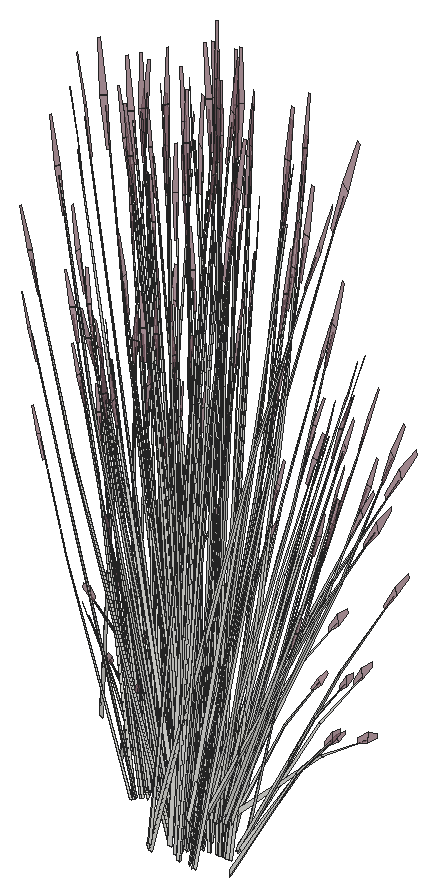
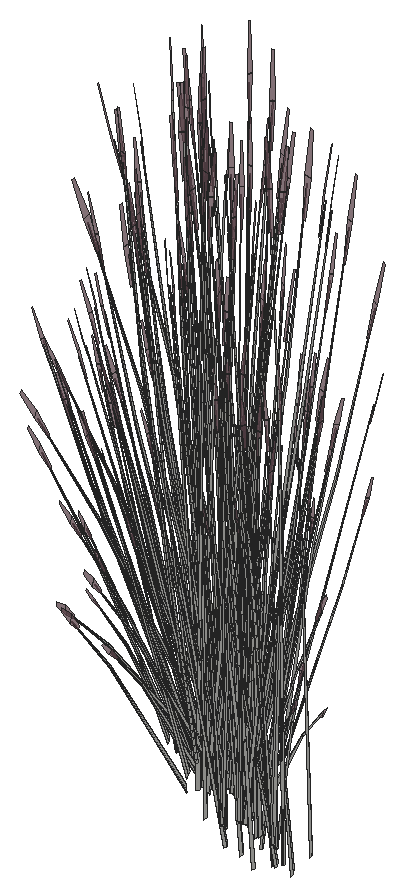
# SketchUp Ruby script. Lengths in inches.
U = 1.inch
M = Sketchup.active_model
def pt(a) = Geom::Point3d.new(a.map { |v| v * U })
def face(e, loops, mat)
  f = e.add_face(loops[0].map { |a| pt(a) })
  loops[1..].each { |l| e.add_face(l.map { |a| pt(a) }).erase! }
  f.material = f.back_material = mat if mat
  f
end
# faces: each face lists its corners as indices into pts; further lists are holes
def faces(e, pts, list, mat = nil) = list.each { |f| face(e, (f[0].is_a?(Array) ? f : [f]).map { |l| l.map { |i| pts[i] } }, mat) }
# xy, xz, yz: faces in a plane at the given z, y or x. An outline is a flat list of corners, or four numbers for a rectangle; further outlines are holes
def ring(l) = l.size == 4 ? [[l[0], l[1]], [l[2], l[1]], [l[2], l[3]], [l[0], l[3]]] : l.each_slice(2).to_a
def flat(e, list, mat, &to3) = list.each { |f| face(e, (f[0].is_a?(Array) ? f : [f]).map { |l| ring(l).map { |u, v| to3.(u, v) } }, mat) }
def xy(e, z, list, mat = nil) = flat(e, list, mat) { |x, y| [x, y, z] }
def xz(e, y, list, mat = nil) = flat(e, list, mat) { |x, z| [x, y, z] }
def yz(e, x, list, mat = nil) = flat(e, list, mat) { |y, z| [x, y, z] }
def lines(e, pts, list) = list.each { |a, b| e.add_line(pt(pts[a]), pt(pts[b])) }
# prism: a flat outline (further loops are holes) pulled along v
def prism(e, loops, v, mat = nil)
  f = face(e, loops, mat); d = Geom::Vector3d.new(v.map { |x| x * U })
  f.pushpull(f.normal.samedirection?(d) ? d.length : -d.length)
end
def box(e, o, s, mat = nil) = prism(e, [[o, [o[0] + s[0], o[1], o[2]], [o[0] + s[0], o[1] + s[1], o[2]], [o[0], o[1] + s[1], o[2]]]], [0, 0, s[2]], mat)
def at(x, y, z, deg = 0) = Geom::Transformation.translation(pt([x, y, z])) * Geom::Transformation.rotation(ORIGIN, Z_AXIS, deg.degrees)
def axes(o, x, y, z) = Geom::Transformation.new([*x, 0, *y, 0, *z, 0, *pt(o).to_a, 1])
def part(name) = M.definitions.add(name)
# library, detail: a bought-in or finely detailed component or shape, given as its bounding box
def library(name, o, s) = part(name).tap { |d| box(d.entities, o, s) }
def detail(e, o, s) = box(e.add_group.entities, o, s)
def put(e, d, t, mat = nil) = e.add_instance(d, t).tap { |i| i.material = mat if mat }
def group(e, t, mat = nil) = e.add_group.tap { |g| g.transformation = t; g.material = mat if mat }.entities
root = M.entities
M.materials.add("LightPink_Translucent").color = [144, 107, 117]
M.materials["LightPink_Translucent"].alpha = 0.75
c1 = part("blade")
p = [[2.15,0.21,22],[0,0.17,0],[0.09,0.45,0],[2.18,0.31,22],[2.29,0.31,22],[0.38,0.45,0],
  [2.48,0.24,33],[2.49,0.24,33],[2.48,0.22,33]]
faces(c1.entities,p,[[0,1,2,3],[4,5,2,3],[6,3,4,7],[8,0,3,6]])
c2 = part("seeds")
p = [[0.3,-0.1,1.38],[-0.01,-0.03,1.59],[-0.01,-0.03,0.03],[0.14,-0.07,-0.07],[0.29,-0.03,3],[0.15,0.01,3.11]]
faces(c2.entities,p,[[0,1,2,3],[1,0,4,5]],"LightPink_Translucent")
c3 = part("blade with seeds")
put(c3.entities,c1,at(0,0,0))
put(c3.entities,c2,axes([2.4,0.25,30.99],[1.5799,-0.05474,1.17369],[-0.12525,1.92788,0.29478],[-0.07173,-0.02425,1.56792]))
put(root,c3,axes([688.24,330.9,391.83],[0,-0.66065,0],[0.81352,0,0],[0,0,1.48949]))
put(root,c3,axes([689.22,329.375,392.06],[-0.60889,-0.28548,0.4121],[0.36394,-0.51192,0],[0.13868,0.06502,1.30728]))
put(root,c3,axes([690.42,331.38,394.13],[0.57168,-0.25217,-0.58968],[0.3186,0.51908,0.07116],[0.27622,-0.05897,0.83415]))
put(root,c3,axes([686.79,331.71,391.71],[-0.67676,-0.09361,-0.51753],[0.14281,-0.57742,-0.13583],[-0.20196,-0.06997,1.14236]))
put(root,c3,axes([687.85,330.48,391.96],[-0.53943,0.51816,0.37976],[-0.64086,-0.4574,0.14902],[0.13005,-0.05171,1.31851]))
put(root,c3,axes([688.44,331.41,391.91],[-0.60515,-0.49144,-0.05089],[0.60552,-0.49174,0],[-0.02113,-0.01716,1.45724]))
put(root,c3,axes([686.92,329.63,392.05],[-0.18794,0.56744,0.14643],[-0.68774,-0.16058,0.29122],[0.1188,-0.00276,1.33138]))
put(root,c3,axes([690.33,331.48,394.19],[-0.54068,-0.15928,0.29394],[0.1577,-0.46469,-0.37948],[0.21769,-0.04261,0.72609]))
put(root,c3,axes([684.67,330.63,393.93],[0.18381,-0.5206,0.39842],[0.60429,0.17802,0.32852],[-0.23764,0.03129,0.82444]))
put(root,c3,axes([686.63,330.09,391.32],[-0.64037,0.22859,1.07011],[-0.20382,-0.65589,0.4158],[0.39323,0.01091,1.21713]))
put(root,c3,axes([688.35,330.26,392.17],[0.12551,-0.50956,0.12018],[0.6132,0.08845,-0.34318],[0.1116,0.05232,1.05198]))
put(root,c3,axes([684.625,330.49,393.93],[-0.23895,-0.38931,0.05337],[0.43573,-0.19055,0.42015],[-0.19208,0.0376,0.64067]))
put(root,c3,axes([687.29,331.47,391.96],[0.82229,0.1203,0.37976],[-0.16734,0.67942,0.14902],[-0.12017,-0.06561,1.31851]))
put(root,c3,axes([691.63,330.98,391.24],[-0.034,-0.08668,1.46364],[0.23582,-0.50706,-0.2236],[0.23788,-0.00729,0.24931]))
put(root,c3,axes([688.09,330.4,392.26],[-0.39083,-0.47924,0.37133],[0.59199,-0.33747,-0.17871],[0.12647,0.0593,1.19224]))
put(root,c3,axes([686.07,332.59,391.68],[-0.15283,-0.49751,-0.25712],[0.60696,-0.14127,0.25712],[-0.12236,-0.05737,1.15348]))
put(root,c3,axes([686.85,332.56,392.05],[0.6991,-0.15154,0.14643],[0.17263,0.56398,0.29122],[-0.06235,-0.08217,1.33138]))
put(root,c3,axes([688.29,330.43,392.21],[0.65687,-0.37907,-0.24149],[0.43681,0.53562,-0.41502],[0.16207,0.0544,1.32557]))
put(root,c3,axes([690.9,331.43,393.76],[0.54068,0.15928,-0.29394],[-0.1577,0.46469,0.37948],[0.21769,-0.04261,0.72609]))
put(root,c3,axes([685.9,332.8,391.67],[-0.60889,-0.28548,-0.4121],[0.36394,-0.51192,0],[-0.13868,-0.06502,1.30728]))
put(root,c3,axes([689.95,329.42,391.67],[0.60889,0.28548,-0.4121],[-0.36394,0.51192,0],[0.13868,0.06502,1.30728]))
put(root,c3,axes([688.79,331.05,391.83],[0.72788,0,0],[0,0.59111,0],[0,0,1.48078]))
put(root,c3,axes([687.56,331.79,392.21],[-0.65687,0.37907,-0.24149],[-0.43681,-0.53562,-0.41502],[-0.16207,-0.0544,1.32557]))
put(root,c3,axes([689,329.66,392.05],[-0.6991,0.15154,0.14643],[-0.17263,-0.56398,0.29122],[0.06235,0.08217,1.33138]))
put(root,c3,axes([689.43,330.85,393.22],[-0.26985,0.01293,1.42242],[0.17902,-0.56047,0.11501],[0.38456,0.03467,0.60807]))
put(root,c3,axes([689.78,329.63,391.68],[0.15283,0.49751,-0.25712],[-0.60696,0.14127,0.25712],[0.12236,0.05737,1.15348]))
put(root,c3,axes([690.82,331.62,393.93],[0.23895,0.38931,0.05337],[-0.43573,0.19055,0.42015],[0.19208,-0.0376,0.64067]))
put(root,c3,axes([688.56,330.75,391.98],[-0.82229,-0.1203,0.40835],[0.16734,-0.67942,0.16024],[0.12017,0.06561,1.41775]))
put(root,c3,axes([690.78,331.48,393.93],[-0.18381,0.5206,0.39842],[-0.60429,-0.17802,0.32852],[0.23764,-0.03129,0.82444]))
put(root,c3,axes([687.9,332.42,391.83],[-0.21227,-0.49226,0],[0.60616,-0.17239,0],[0,0,1.28128]))
put(root,c3,axes([687.49,331.96,392.17],[-0.12551,0.50956,0.12018],[-0.6132,-0.08845,-0.34318],[-0.1116,-0.05232,1.05198]))
put(root,c3,axes([685.12,330.63,394.19],[0.54068,0.15928,0.29394],[-0.1577,0.46469,-0.37948],[-0.21769,0.04261,0.72609]))
put(root,c3,axes([688.69,332.35,391.8125],[0.68303,-0.19373,-0.15934],[0.24001,0.55805,0.00007],[0.07539,-0.02141,1.44335]))
put(root,c3,axes([688.93,332.59,392.05],[0.18794,-0.56744,0.14643],[0.68774,0.16058,0.29122],[-0.1188,0.00276,1.33138]))
put(root,c3,axes([688.77,331.3,391.84],[0.45414,0.3688,0],[-0.45414,0.3688,0],[0,0,1.40491]))
put(root,c3,axes([690,331.14,392.05],[-0.51116,-0.4159,0.14643],[0.51512,-0.4034,0.29122],[-0.05645,0.08494,1.33138]))
put(root,c3,axes([689.06,330.51,391.71],[0.67676,0.09361,-0.51753],[-0.14281,0.57742,-0.13583],[0.20196,0.06997,1.14236]))
put(root,c3,axes([692.05,331.52,392.3],[-0.40197,0.09426,0.95334],[0.18921,-0.38956,0.70045],[0.21325,0.02666,0.20998]))
put(root,c3,axes([687.75,332.65,391.82],[-0.65588,-0.25634,0],[0.31565,-0.53263,0],[0,0,1.35047]))
put(root,c3,axes([688.29,331.96,392.05],[-0.63528,-0.45956,-0.20909],[0.53456,-0.51604,0.45758],[-0.17107,0.05376,1.39619]))
put(root,c3,axes([686.62,332.84,392.06],[0.60889,0.28548,0.4121],[-0.36394,0.51192,0],[-0.13868,-0.06502,1.30728]))
put(root,c3,axes([688.77,330.87,392.26],[0.31565,-0.51449,0.37133],[0.65588,0.24761,-0.17871],[0,0.1186,1.19224]))
put(root,c3,axes([691.86,333.17,393.91],[-0.05883,-0.04999,1.47228],[0.12868,-0.53581,-0.13912],[0.23172,-0.03423,0.26054]))
put(root,c3,axes([688.65,331.16,391.9],[0,0.66033,-0.04679],[-0.81352,0,0],[0,0.02075,1.48875]))
put(root,c3,axes([684.89,330.48,394.18],[0.32734,0.51701,-0.10093],[-0.58097,0.25407,-0.56021],[-0.24483,0.06821,0.85122]))
put(root,c3,axes([688.71,330.7,391.83],[0.39083,0.47924,-0.37133],[-0.59199,0.33747,0.17871],[0.12647,0.0593,1.19224]))
put(root,c3,axes([691.35,332.72,393.26],[-0.12452,-0.47997,-0.02898],[0.58854,-0.11034,-0.1314],[0.1229,0.03043,0.43341]))
put(root,c3,axes([686.27,333.14,391.97],[-0.40676,0.57214,0],[-0.68052,-0.31907,-0.42834],[-0.15499,-0.07267,1.3588]))
put(root,c3,axes([689.82,332.71,394.18],[0.03484,-0.58066,-0.10093],[0.65957,0.01587,-0.56021],[0.25402,0.04034,0.85122]))
put(root,c3,axes([690.42,331.16,392.06],[0,-0.57097,0.4121],[0.72788,0,0],[0,0.13004,1.30728]))
put(root,c3,axes([688.6,331.58,392.26],[0.70648,-0.03525,0.37133],[0.06389,0.58508,-0.17871],[-0.12647,0.0593,1.19224]))
put(root,c3,axes([689.04,330.99,392.17],[0.60616,-0.16651,0.12018],[0.21227,0.47548,-0.34318],[0,0.10465,1.05198]))
put(root,c3,axes([689.72,332.48,394.19],[-0.37017,-0.35748,0.29394],[0.42268,-0.3384,-0.37948],[0.21476,0.05149,0.72609]))
put(root,c3,axes([687.97,331.87,391.83],[-0.70648,0.03525,-0.37133],[-0.06389,-0.58508,0.17871],[-0.12647,0.0593,1.19224]))
put(root,c3,axes([691.29,332.15,392.15],[-0.15668,-0.14043,1.18691],[0.20386,-0.46454,-0.25526],[0.31701,0.06293,0.50747]))
put(root,c3,axes([681.05,337.49,392.15],[-0.18493,0.11557,1.18691],[-0.55384,-0.20228,-0.25526],[0.10266,-0.25157,0.50747]))
put(root,c3,axes([688.49,332.66,391.83],[0.65588,0.25634,0],[-0.31565,0.53263,0],[0,0,1.45212]))
put(root,c3,axes([690.4,332.36,393.91],[0.13956,-0.00966,1.45204],[0.38281,-0.44358,-0.22964],[0.24825,0.05855,0.11645]))
put(root,c3,axes([688.76,333.22,391.82],[-0.40169,-0.57414,-0.04268],[0.68052,-0.31907,0.42834],[-0.16769,0.05466,1.35813]))
put(root,c3,axes([688.61,331.83,392.17],[0.48065,0.34305,0.12018],[-0.40092,0.38703,-0.34318],[-0.1116,0.05232,1.05198]))
put(root,c3,axes([684.82,331.92,393.93],[-0.16135,-0.52549,0.39842],[0.63294,-0.0912,0.32852],[-0.18654,0.12359,0.82444]))
put(root,c3,axes([684.69,331.82,393.93],[-0.44663,-0.24013,0.05337],[0.26003,-0.34195,0.42015],[-0.14319,0.11055,0.64067]))
put(root,c3,axes([681.5,338.35,394.13],[0.01693,-0.52814,-0.58968],[0.71285,0.03547,0.07116],[0.07523,-0.22375,0.83415]))
put(root,c3,axes([689.86,332.43,394.13],[0.65035,0.01375,-0.58968],[-0.04368,0.5789,0.07116],[0.27552,0.06109,0.83415]))
put(root,c3,axes([682.49,337.52,393.91],[-0.00628,-0.11364,1.45204],[-0.53042,-0.32843,-0.22964],[0.08201,-0.19909,0.11645]))
put(root,c3,axes([676.63,338.08,393.22],[-0.12114,0.19625,1.42242],[-0.50818,-0.40613,0.11501],[0.22925,-0.25313,0.60807]))
put(root,c3,axes([680.7,338.08,393.22],[-0.12114,0.19625,1.42242],[-0.50818,-0.40613,0.11501],[0.22925,-0.25313,0.60807]))
put(root,c3,axes([682.35,337.11,393.91],[-0.06607,0.04361,1.47228],[-0.64734,-0.14714,-0.13912],[-0.02343,-0.19032,0.26054]))
put(root,c3,axes([689.125,332.89,392.06],[0.60889,-0.28548,0.4121],[0.36394,0.51192,0],[-0.13868,0.06502,1.30728]))
put(root,c3,axes([688.26,332.44,391.9],[0.28286,0.65594,-0.0499],[-0.80821,0.22985,0],[0.00988,0.02291,1.42904]))
put(root,c3,axes([688.57,333.15,391.68],[-0.60696,-0.14127,-0.25712],[0.15283,-0.49751,0.25712],[-0.12236,0.05737,1.15348]))
put(root,c3,axes([680.37,336.57,392.3],[0.08346,0.33295,0.95334],[-0.46298,-0.1844,0.70045],[0.04982,-0.17048,0.20998]))
put(root,c3,axes([685.21,331.75,394.19],[0.56631,-0.0816,0.29394],[0.14954,0.46647,-0.37948],[-0.16229,0.12529,0.72609]))
put(root,c3,axes([690.92,331.25,391.97],[0.81352,0,0],[0,0.63814,-0.42834],[0,0.14534,1.3588]))
put(root,c3,axes([681.36,338.17,393.89],[-0.46573,-0.38364,-0.42412],[0.49199,-0.33598,-0.32852],[0.07086,-0.19492,0.81151]))
put(root,c3,axes([690.59,331.58,391.83],[-0.81312,-0.00457,-0.0413],[0,-0.63814,0.41452],[-0.02555,0.14527,1.31432]))
put(root,c3,axes([688.83,331.03,392.21],[0.73268,0.27244,-0.24149],[-0.35279,0.57501,-0.41502],[0.02303,0.14118,1.32557]))
put(root,c3,axes([683.72,333.14,392.3],[0.27113,-0.25877,0.95334],[0.10699,0.40966,0.70045],[-0.19594,0.07335,0.20998]))
put(root,c3,axes([690.25,332.67,393.76],[0.37017,0.35748,-0.29394],[-0.42268,0.3384,0.37948],[0.21476,0.05149,0.72609]))
put(root,c3,axes([690.42,331.67,391.68],[-0.45414,0.35624,-0.25712],[-0.45414,-0.35624,0.25712],[0,0.11474,1.15348]))
put(root,c3,axes([688.47,331.71,392.21],[0.07581,0.65151,-0.24149],[-0.7896,0.03939,-0.41502],[-0.13904,0.08678,1.32557]))
put(root,c3,axes([690.06,332.8,393.93],[-0.03276,0.43418,0.05337],[-0.49468,-0.0119,0.42015],[0.18949,0.04543,0.64067]))
put(root,c3,axes([688.76,331.45,391.83],[-0.31565,0.51449,-0.37133],[-0.65588,-0.24761,0.17871],[0,0.1186,1.19224]))
put(root,c3,axes([684.74,332.03,393.76],[-0.56631,0.0816,-0.29394],[-0.14954,-0.46647,0.37948],[-0.16229,0.12529,0.72609]))
put(root,c3,axes([690.1,332.67,393.93],[-0.47971,0.37622,0.39842],[-0.41372,-0.39954,0.32852],[0.22506,0.0694,0.82444]))
put(root,c3,axes([680.34,337.6,393.93],[0.64106,0.14927,0.39842],[-0.21921,0.49074,0.32852],[-0.03852,-0.19299,0.82444]))
put(root,c3,axes([681.84,338.37,394.18],[-0.71502,-0.02829,-0.10093],[0.01954,-0.53563,-0.56021],[0.04967,-0.20629,0.85122]))
put(root,c3,axes([681.79,338.03,393.76],[0.4402,-0.30062,-0.29394],[0.41671,0.34326,0.37948],[0.0634,-0.1744,0.72609]))
put(root,c3,axes([683.92,333.07,394.6875],[0.5741,0.15241,-0.05385],[-0.1766,0.46909,-0.24415],[-0.0939,0.07122,0.8053]))
put(root,c3,axes([687.99,332.21,391.71],[-0.43821,0.42916,-0.51753],[-0.54436,-0.38915,-0.13583],[-0.1756,0.10706,1.14236]))
put(root,c3,axes([688.58,333.1,394.19],[-0.10048,-0.4599,0.29394],[0.5744,-0.12144,-0.37948],[0.15428,0.13179,0.72609]))
put(root,c3,axes([688.77,332.93,391.93],[0.81449,0.18558,0.25528],[-0.20377,0.66335,-0.30288],[-0.13481,0.08302,1.36855]))
put(root,c3,axes([688.71,333.375,391.67],[-0.60889,0.28548,-0.4121],[-0.36394,-0.51192,0],[-0.13868,0.06502,1.30728]))
put(root,c3,axes([690.74,331.6875,391.67],[0,0.57097,-0.4121],[-0.72788,0,0],[0,0.13004,1.30728]))
put(root,c3,axes([688.92,331.75,393.22],[-0.24166,-0.09837,1.42242],[0.50011,-0.41269,0.11501],[0.3117,0.18617,0.60807]))
put(root,c3,axes([688.96,330.46,393.71],[-0.56218,-0.29666,1.14775],[0.59361,-0.46189,0.49522],[0.18138,0.27836,1.10941]))
put(root,c3,axes([684.91,331.71,394.18],[0.60181,0.31483,-0.10093],[-0.34671,0.45593,-0.56021],[-0.17003,0.15849,0.85122]))
put(root,c3,axes([689.8125,332.87,392.3],[-0.36631,-0.16417,0.95334],[0.47299,-0.16681,0.70045],[0.12758,0.1413,0.20998]))
put(root,c3,axes([688.53,333.34,394.18],[0.38768,-0.48872,-0.10093],[0.56143,0.28156,-0.56021],[0.19516,0.13808,0.85122]))
put(root,c3,axes([678.27,337.85,391.24],[-0.09738,-0.04498,1.46364],[-0.25012,-0.50252,-0.2236],[0.16873,-0.13637,0.24931]))
put(root,c3,axes([682.34,337.85,391.24],[-0.09738,-0.04498,1.46364],[-0.25012,-0.50252,-0.2236],[0.16873,-0.13637,0.24931]))
put(root,c3,axes([685.72,331.57,393.22],[0.1625,-0.17544,1.42242],[0.41029,0.47354,0.11501],[-0.28141,0.21565,0.60807]))
put(root,c3,axes([685.21,332.08,393.89],[0.16713,0.52135,-0.42412],[-0.63294,0.0912,-0.32852],[-0.18138,0.14003,0.81151]))
put(root,c3,axes([681.79,338.14,393.93],[0.46327,0.38957,0.39842],[-0.49199,0.33598,0.32852],[0.08546,-0.18277,0.82444]))
put(root,c3,axes([685.97,332.68,394.19],[0.4402,-0.30062,0.29394],[0.41671,0.34326,-0.37948],[-0.0634,0.1744,0.72609]))
put(root,c3,axes([689.27,333.29,391.97],[0.40676,0.57214,0],[-0.68052,0.31907,-0.42834],[-0.15499,0.07267,1.3588]))
put(root,c3,axes([681.96,338.18,393.93],[0.53464,0.0266,0.05337],[-0.01466,0.40172,0.42015],[0.05594,-0.15388,0.64067]))
put(root,c3,axes([688.02,333.74,393.91],[0.00193,-0.06913,1.47228],[0.55753,-0.30498,-0.13912],[0.19366,0.10886,0.26054]))
put(root,c3,axes([689.92,333.48,391.24],[0.0474,-0.08243,1.46364],[0.59674,-0.24277,-0.2236],[0.18092,0.12565,0.24931]))
put(root,c3,axes([688.92,331.02,392.36],[-0.01777,-0.53759,1.17256],[0.80434,0.13935,0.49647],[-0.19024,0.29416,1.1068]))
put(root,c3,axes([689.13,331.61,391.74],[0.23855,0.52277,-0.57446],[-0.68718,0.18827,-0.15077],[0.02637,0.17702,1.26801]))
put(root,c3,axes([685.57,332.95,393.93],[-0.53464,-0.0266,0.05337],[0.01466,-0.40172,0.42015],[-0.05594,0.15388,0.64067]))
put(root,c3,axes([684.44,333.41,391.24],[0.08727,0.05704,1.46364],[0.14797,0.52853,-0.2236],[-0.19341,0.11271,0.24931]))
put(root,c3,axes([681.5625,338.45,394.19],[-0.4402,0.30062,0.29394],[-0.41671,-0.34326,-0.37948],[0.0634,-0.1744,0.72609]))
put(root,c3,axes([685.74,332.99,393.93],[-0.46327,-0.38957,0.39842],[0.49199,-0.33598,0.32852],[-0.08546,0.18277,0.82444]))
put(root,c3,axes([688.99,333.1,393.89],[0.64198,-0.13573,-0.42412],[0.1123,0.514,-0.32852],[0.17243,0.1473,0.81151]))
put(root,c3,axes([678.27,339.26,394.13],[0.33983,-0.45051,-0.58968],[0.59551,0.32017,0.07116],[0.20291,-0.16322,0.83415]))
put(root,c3,axes([682.34,339.26,394.13],[0.33983,-0.45051,-0.58968],[0.59551,0.32017,0.07116],[0.20291,-0.16322,0.83415]))
put(root,c3,axes([678.67,337.95,391.97],[-0.40676,-0.57214,0],[0.68052,-0.31907,-0.42834],[0.15499,-0.07267,1.3588]))
put(root,c3,axes([678.25,339.05,393.89],[-0.16713,-0.52135,-0.42412],[0.63294,-0.0912,-0.32852],[0.18138,-0.14003,0.81151]))
put(root,c3,axes([682.32,339.05,393.89],[-0.16713,-0.52135,-0.42412],[0.63294,-0.0912,-0.32852],[0.18138,-0.14003,0.81151]))
put(root,c3,axes([687.2,333.17,394.19],[0.19614,-0.43908,0.29394],[0.57222,0.12807,-0.37948],[0.05247,0.17678,0.72609]))
put(root,c3,axes([689.87,333.62,392.21],[-0.4172,-0.01791,0.872],[0.27552,-0.38032,0.48145],[0.16481,0.13512,0.68401]))
put(root,c3,axes([678.55,339.43,394.18],[-0.60181,-0.31483,-0.10093],[0.34671,-0.45593,-0.56021],[0.17003,-0.15849,0.85122]))
put(root,c3,axes([682.62,339.43,394.18],[-0.60181,-0.31483,-0.10093],[0.34671,-0.45593,-0.56021],[0.17003,-0.15849,0.85122]))
put(root,c3,axes([688.67,333.52,393.93],[-0.29569,0.36271,0.05337],[-0.42107,-0.21117,0.42015],[0.13613,0.11629,0.64067]))
put(root,c3,axes([687.97,334.74,394.6875],[0.44958,-0.32756,-0.05385],[0.41194,0.35875,-0.24415],[0.029,0.10165,0.8053]))
put(root,c3,axes([688.79,333.42,393.93],[-0.64708,0.13103,0.39842],[-0.1123,-0.514,0.32852],[0.15218,0.15149,0.82444]))
put(root,c3,axes([679.22,337.86,391.67],[0.60889,-0.28548,-0.4121],[0.36394,0.51192,0],[0.13868,-0.06502,1.30728]))
put(root,c3,axes([685.6,332,393.22],[0.12114,-0.19625,1.42242],[0.50818,0.40613,0.11501],[-0.22925,0.25313,0.60807]))
put(root,c3,axes([678.76,338.85,392.15],[-0.23242,-0.01691,1.18691],[-0.23811,-0.45367,-0.25526],[0.28553,-0.12834,0.50747]))
put(root,c3,axes([682.83,338.85,392.15],[-0.23242,-0.01691,1.18691],[-0.23811,-0.45367,-0.25526],[0.28553,-0.12834,0.50747]))
put(root,c3,axes([680.04,339.29,393.91],[-0.08498,-0.00434,1.47228],[-0.35287,-0.46464,-0.13912],[0.14171,-0.15278,0.26054]))
put(root,c3,axes([684.1,339.29,393.91],[-0.08498,-0.00434,1.47228],[-0.35287,-0.46464,-0.13912],[0.14171,-0.15278,0.26054]))
put(root,c3,axes([688.51,332.7,392.15],[0.01148,-0.18927,1.18691],[0.54864,-0.21141,-0.25526],[0.16937,0.22654,0.50747]))
put(root,c3,axes([679.94,339.03,391.71],[0.43821,-0.42916,-0.51753],[0.54436,0.38915,-0.13583],[0.1756,-0.10706,1.14236]))
